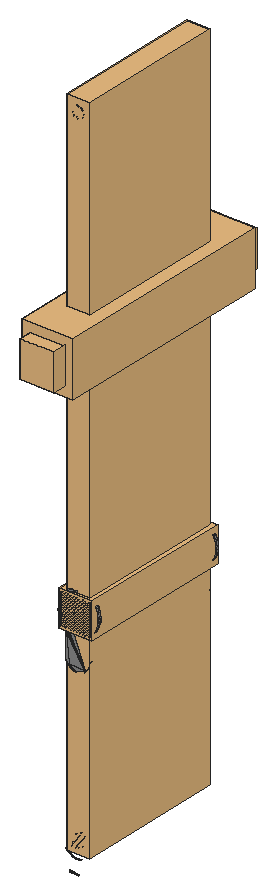
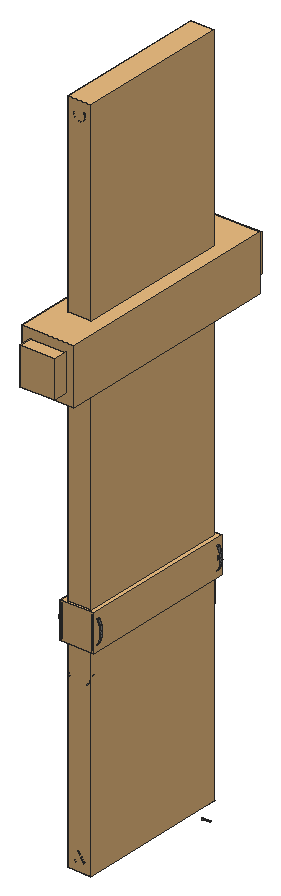
# SketchUp Ruby script. Lengths in inches.
U = 1.inch
M = Sketchup.active_model
def pt(a) = Geom::Point3d.new(a.map { |v| v * U })
def face(e, loops, mat)
  f = e.add_face(loops[0].map { |a| pt(a) })
  loops[1..].each { |l| e.add_face(l.map { |a| pt(a) }).erase! }
  f.material = f.back_material = mat if mat
  f
end
# faces: each face lists its corners as indices into pts; further lists are holes
def faces(e, pts, list, mat = nil) = list.each { |f| face(e, (f[0].is_a?(Array) ? f : [f]).map { |l| l.map { |i| pts[i] } }, mat) }
# xy, xz, yz: faces in a plane at the given z, y or x. An outline is a flat list of corners, or four numbers for a rectangle; further outlines are holes
def ring(l) = l.size == 4 ? [[l[0], l[1]], [l[2], l[1]], [l[2], l[3]], [l[0], l[3]]] : l.each_slice(2).to_a
def flat(e, list, mat, &to3) = list.each { |f| face(e, (f[0].is_a?(Array) ? f : [f]).map { |l| ring(l).map { |u, v| to3.(u, v) } }, mat) }
def xy(e, z, list, mat = nil) = flat(e, list, mat) { |x, y| [x, y, z] }
def xz(e, y, list, mat = nil) = flat(e, list, mat) { |x, z| [x, y, z] }
def yz(e, x, list, mat = nil) = flat(e, list, mat) { |y, z| [x, y, z] }
def lines(e, pts, list) = list.each { |a, b| e.add_line(pt(pts[a]), pt(pts[b])) }
# prism: a flat outline (further loops are holes) pulled along v
def prism(e, loops, v, mat = nil)
  f = face(e, loops, mat); d = Geom::Vector3d.new(v.map { |x| x * U })
  f.pushpull(f.normal.samedirection?(d) ? d.length : -d.length)
end
def box(e, o, s, mat = nil) = prism(e, [[o, [o[0] + s[0], o[1], o[2]], [o[0] + s[0], o[1] + s[1], o[2]], [o[0], o[1] + s[1], o[2]]]], [0, 0, s[2]], mat)
def at(x, y, z, deg = 0) = Geom::Transformation.translation(pt([x, y, z])) * Geom::Transformation.rotation(ORIGIN, Z_AXIS, deg.degrees)
def axes(o, x, y, z) = Geom::Transformation.new([*x, 0, *y, 0, *z, 0, *pt(o).to_a, 1])
def part(name) = M.definitions.add(name)
# library, detail: a bought-in or finely detailed component or shape, given as its bounding box
def library(name, o, s) = part(name).tap { |d| box(d.entities, o, s) }
def detail(e, o, s) = box(e.add_group.entities, o, s)
def put(e, d, t, mat = nil) = e.add_instance(d, t).tap { |i| i.material = mat if mat }
def group(e, t, mat = nil) = e.add_group.tap { |g| g.transformation = t; g.material = mat if mat }.entities
root = M.entities
M.materials.add("Material \#1").color = [140, 140, 140]
c1 = library("3DGeom~14_Defintion",[-102.17,352.37,-727.27],[204.35,204.35,1000])
c2 = library("3DGeom~4_Defintion",[-18.02,-499.97,-221.16],[36.04,1000,262.12])
c3 = part("3DGeom~5_Defintion")
xy(c3.entities,-225.24,[[-0.79,-499.98,-2.33,-499.64,7.45,-496.14],[-0.79,-499.98,7.45,-496.14,1.58,-499.88],[1.58,-499.88,7.45,-496.14,3.84,-499.16],[-2.33,-499.64,7.4,-485.75,7.45,-496.14],[3.84,-499.16,7.45,-496.14,5.85,-497.89],
  [7.45,-496.14,7.4,-485.75,8.24,-487.08],[7.45,-496.14,8.24,-487.08,8.96,-489.34],[7.45,-496.14,8.96,-489.34,9.0625,-491.71],[7.45,-496.14,9.0625,-491.71,8.55,-494.03],[-7.4,-496.08,-8.24,-494.76,2.32,-482.2],
  [-8.24,-494.76,-8.96,-492.5,2.32,-482.2],[-8.96,-492.5,-9.0625,-490.125,2.32,-482.2],[-9.0625,-490.125,-8.55,-487.81,2.32,-482.2],[-8.55,-487.81,-7.45,-485.7,2.32,-482.2],[-7.45,-485.7,-5.85,-483.95,2.32,-482.2],
  [-5.85,-483.95,-3.84,-482.68,2.32,-482.2],[-3.84,-482.68,-1.58,-481.96,2.32,-482.2],[2.32,-482.2,-1.58,-481.96,0.79,-481.86],[0,481.82,-2.35,482.13,-6.92,496.71],[0,481.82,-6.92,496.71,1.55,482.04],
  [-2.35,482.13,-4.55,483.04,-6.92,496.71],[-4.55,483.04,-6.43,484.49,-6.92,496.71],[-6.43,484.49,-7.88,486.37,-6.92,496.71],[6.92,485.12,-1.55,499.8125,7.88,495.47],[6.92,485.12,7.88,495.47,7.88,486.37],
  [-7.88,486.37,-8.79,488.57,-6.92,496.71],[7.88,486.37,7.88,495.47,8.79,488.57],[-8.79,488.57,-9.1,490.92,-6.92,496.71],[8.79,488.57,7.88,495.47,9.1,490.92],[-9.1,490.92,-8.79,493.28,-6.92,496.71],
  [9.1,490.92,7.88,495.47,8.79,493.28],[-8.79,493.28,-7.88,495.47,-6.92,496.71],[7.88,495.47,-1.55,499.8125,0,500.02],[7.88,495.47,0,500.02,2.35,499.71],[7.88,495.47,2.35,499.71,4.55,498.8],
  [7.88,495.47,4.55,498.8,6.43,497.35]],"Material \#1")
xy(c3.entities,-221.57,[[-2.33,-499.64,-5.22,-498.37,7.4,-485.75],[-5.22,-498.37,-7.4,-496.08,5.22,-483.47],[-5.22,-498.37,5.22,-483.47,7.4,-485.75],[-7.4,-496.08,2.32,-482.2,5.22,-483.47],[1.55,482.04,-6.92,496.71,-4.55,498.8],
  [1.55,482.04,-4.55,498.8,4.55,483.04],[4.55,483.04,-4.55,498.8,-1.55,499.8125],[4.55,483.04,-1.55,499.8125,6.92,485.12]],"Material \#1")
xy(c3.entities,38.05,[[-2.33,-499.64,7.4,-485.75,-5.22,-498.37],[-5.22,-498.37,5.22,-483.47,-7.4,-496.08],[-5.22,-498.37,7.4,-485.75,5.22,-483.47],[-7.4,-496.08,5.22,-483.47,2.32,-482.2],[1.55,482.04,-4.55,498.8,-6.92,496.71],
  [1.55,482.04,4.55,483.04,-4.55,498.8],[4.55,483.04,-1.55,499.8125,-4.55,498.8],[4.55,483.04,6.92,485.12,-1.55,499.8125]],"Material \#1")
xy(c3.entities,41.72,[[-0.79,-499.98,7.45,-496.14,-2.33,-499.64],[-0.79,-499.98,1.58,-499.88,7.45,-496.14],[1.58,-499.88,3.84,-499.16,7.45,-496.14],[-2.33,-499.64,7.45,-496.14,7.4,-485.75],[3.84,-499.16,5.85,-497.89,7.45,-496.14],
  [7.45,-496.14,8.24,-487.08,7.4,-485.75],[7.45,-496.14,8.55,-494.03,9.0625,-491.71],[7.45,-496.14,8.96,-489.34,8.24,-487.08],[7.45,-496.14,9.0625,-491.71,8.96,-489.34],[-7.4,-496.08,2.32,-482.2,-8.24,-494.76],
  [-8.24,-494.76,2.32,-482.2,-8.96,-492.5],[-8.96,-492.5,2.32,-482.2,-9.0625,-490.125],[-9.0625,-490.125,2.32,-482.2,-8.55,-487.81],[-8.55,-487.81,2.32,-482.2,-7.45,-485.7],[-7.45,-485.7,2.32,-482.2,-5.85,-483.95],
  [-5.85,-483.95,2.32,-482.2,-3.84,-482.68],[-3.84,-482.68,2.32,-482.2,-1.58,-481.96],[2.32,-482.2,0.79,-481.86,-1.58,-481.96],[0,481.82,-6.92,496.71,-2.35,482.13],[0,481.82,1.55,482.04,-6.92,496.71],
  [-2.35,482.13,-6.92,496.71,-4.55,483.04],[-4.55,483.04,-6.92,496.71,-6.43,484.49],[-6.43,484.49,-6.92,496.71,-7.88,486.37],[6.92,485.12,7.88,495.47,-1.55,499.8125],[6.92,485.12,7.88,486.37,7.88,495.47],
  [-7.88,486.37,-6.92,496.71,-8.79,488.57],[7.88,486.37,8.79,488.57,7.88,495.47],[-8.79,488.57,-6.92,496.71,-9.1,490.92],[8.79,488.57,9.1,490.92,7.88,495.47],[-9.1,490.92,-6.92,496.71,-8.79,493.28],
  [9.1,490.92,8.79,493.28,7.88,495.47],[-8.79,493.28,-6.92,496.71,-7.88,495.47],[7.88,495.47,0,500.02,-1.55,499.8125],[7.88,495.47,2.35,499.71,0,500.02],[7.88,495.47,4.55,498.8,2.35,499.71],
  [7.88,495.47,6.43,497.35,4.55,498.8]],"Material \#1")
c4 = library("3DGeom~1_Defintion",[-60.87,347.29,-704.08],[121.74,121.75,1000])
c5 = part("3DGeom~10_Defintion")
yz(c5.entities,-68.96,[[-797.08,-844.83,-797.08,-827.59,-922.41,-827.59],[-922.41,-844.83,-797.08,-844.83,-922.41,-827.59]],"Material \#1")
yz(c5.entities,68.97,[[-922.41,-844.83,-797.08,-827.59,-797.08,-844.83],[-922.41,-844.83,-922.41,-827.59,-797.08,-827.59],[-797.08,137.93,-922.41,155.17,-797.08,155.17],[-922.41,137.93,-922.41,155.17,-797.08,137.93]],"Material \#1")
p = [[-15.8,-989.55,-844.83],[-15.8,-989.55,-827.59],[0,-991.38,-827.59],[0,-991.38,-844.83],[15.8,-989.55,-827.59],[15.8,-989.55,-844.83],
  [-30.32,-984.36,-844.83],[-30.32,-984.36,-827.59],[30.31,-984.36,-827.59],[30.31,-984.36,-844.83],[-43.12,-976.21,-844.83],[-43.12,-976.21,-827.59],
  [43.12,-976.21,-827.59],[43.12,-976.21,-844.83],[-53.81,-965.53,-844.83],[-53.81,-965.53,-827.59],[53.8,-965.53,-827.59],[53.8,-965.53,-844.83],
  [-61.95,-952.73,-844.83],[-61.95,-952.73,-827.59],[53.8,-965.53,-827.59],[61.95,-952.73,-827.59],[61.95,-952.73,-844.83],[-67.15,-938.21,-844.83],
  [-67.15,-938.21,-827.59],[67.14,-938.21,-827.59],[67.14,-938.21,-844.83],[-68.96,-922.41,-844.83],[-68.96,-922.41,-827.59],[67.14,-938.21,-827.59],
  [68.97,-922.41,-827.59],[68.97,-922.41,-844.83],[-69.1,-794.86,-844.83],[-69.1,-794.86,-827.59],[-68.96,-797.08,-827.59],[-68.96,-797.08,-844.83],
  [68.97,-797.08,-844.83],[68.97,-797.08,-827.59],[69.11,-794.71,-827.59],[69.11,-794.71,-844.83],[-69.48,-792.73,-844.83],[-69.48,-792.73,-827.59],
  [69.53,-792.51,-827.59],[69.53,-792.51,-844.83],[-70.14,-790.6875,-844.83],[-70.14,-790.6875,-827.59],[70.24,-790.48,-827.59],[70.24,-790.48,-844.83],
  [-71.08,-788.73,-844.83],[-71.08,-788.73,-827.59],[71.22,-788.57,-827.59],[71.22,-788.57,-844.83],[-72.32,-786.86,-844.83],[-72.32,-786.86,-827.59],
  [72.47,-786.78,-827.59],[72.47,-786.78,-844.83],[-73.8,-785.17,-844.83],[-73.8,-785.17,-827.59],[74,-785.04,-827.59],[74,-785.04,-844.83],
  [-75.96,-783.21,-844.83],[-75.96,-783.21,-827.59],[74,-785.04,-827.59],[75.76,-783.39,-827.59],[75.76,-783.39,-844.83],[86.625,-772.95,-827.59],
  [86.61,-772.96,-844.83],[-86.89,-773.25,-844.83],[-86.89,-773.25,-827.59],[-75.96,-783.21,-844.83],[-96.66,-761.8,-844.83],[-96.66,-761.8,-827.59],
  [86.625,-772.95,-827.59],[86.63,-772.94,-844.83],[86.61,-772.96,-844.83],[86.625,-772.95,-827.59],[86.62,-772.95,-827.59],[86.62,-772.95,-827.59],
  [96.31,-761.375,-827.59],[96.31,-761.375,-844.83],[86.63,-772.94,-844.83],[86.625,-772.95,-827.59],[86.62,-772.95,-827.59],[-104.96,-749.18,-844.83],
  [-104.96,-749.18,-827.59],[-96.66,-761.8,-827.59],[-96.66,-761.8,-844.83],[96.31,-761.375,-827.59],[104.62,-748.77,-827.59],[104.62,-748.77,-844.83],
  [-111.64,-735.52,-844.83],[-111.64,-735.52,-827.59],[111.39,-735.21,-827.59],[111.39,-735.21,-844.83],[-116.49,-721.23,-844.83],[-116.49,-721.23,-827.59],
  [116.4375,-720.78,-827.59],[116.4375,-720.78,-844.83],[-119.64,-705.62,-844.83],[-119.64,-705.62,-827.59],[119.6,-705.57,-827.59],[119.6,-705.57,-844.83],
  [-120.6875,-689.65,-844.83],[-120.6875,-689.65,-827.59],[120.69,-689.65,-827.59],[120.69,-689.65,-844.83],[-117.5,-662,-844.83],[-117.5,-662,-827.59],
  [117.5,-662,-827.59],[117.5,-662,-844.83],[-108.41,-636.61,-844.83],[-108.41,-636.61,-827.59],[117.5,-662,-844.83],[108.41,-636.61,-827.59],
  [108.41,-636.61,-844.83],[-93.91,-613.95,-844.83],[-93.91,-613.95,-827.59],[-108.41,-636.61,-827.59],[108.41,-636.61,-844.83],[94.16,-614.19,-827.59],
  [94.16,-614.19,-844.83],[94.16,-614.19,-827.59],[75.46,-595.5,-827.59],[75.46,-595.5,-844.83],[-75.46,-595.5,-844.83],[-75.46,-595.5,-827.59],
  [-93.91,-613.95,-827.59],[-93.91,-613.95,-827.59],[-93.91,-613.95,-844.83],[-53.05,-581.24,-844.83],[-53.05,-581.24,-827.59],[-75.46,-595.5,-827.59],
  [-75.46,-595.5,-844.83],[53.05,-581.24,-827.59],[53.05,-581.24,-844.83],[-27.65,-572.16,-844.83],[-27.65,-572.16,-827.59],[-53.05,-581.24,-827.59],
  [-53.05,-581.24,-844.83],[27.66,-572.16,-827.59],[27.66,-572.16,-844.83],[0,-568.97,-844.83],[0,-568.97,-827.59],[-27.65,-572.16,-827.59],
  [-27.65,-572.16,-844.83],[0,-568.97,-844.83],[-15.8,-989.55,155.17],[0,-991.38,155.17],[0,-991.38,137.93],[-15.8,-989.55,137.93],
  [15.8,-989.55,155.17],[15.8,-989.55,137.93],[-30.32,-984.36,155.17],[-30.32,-984.36,137.93],[30.31,-984.36,155.17],[30.31,-984.36,137.93],
  [-43.125,-976.22,155.17],[-43.125,-976.22,137.93],[43.12,-976.22,155.17],[43.12,-976.22,137.93],[-53.81,-965.53,155.17],[-53.81,-965.53,137.93],
  [53.8,-965.53,155.17],[53.8,-965.53,137.93],[-61.96,-952.73,155.17],[-61.95,-952.73,137.93],[61.95,-952.73,155.17],[61.95,-952.73,137.93],
  [53.8,-965.53,137.93],[-67.15,-938.21,155.17],[-67.15,-938.21,137.93],[67.14,-938.21,155.17],[67.14,-938.21,137.93],[-68.96,-922.41,155.17],
  [-68.96,-922.41,137.93],[68.97,-922.41,155.17],[68.97,-922.41,137.93],[67.14,-938.21,137.93],[-68.97,-797.08,155.17],[-68.97,-797.08,137.93],
  [-69.1,-794.86,155.17],[-69.1,-794.86,137.93],[68.97,-797.08,155.17],[69.11,-794.71,155.17],[69.11,-794.71,137.93],[68.97,-797.08,137.93],
  [-69.48,-792.73,155.17],[-69.48,-792.73,137.93],[69.53,-792.51,155.17],[69.53,-792.51,137.93],[-70.14,-790.6875,155.17],[-70.14,-790.6875,137.93],
  [70.24,-790.48,155.17],[70.24,-790.48,137.93],[-71.08,-788.73,155.17],[-71.08,-788.73,137.93],[71.22,-788.57,155.17],[71.22,-788.57,137.93],
  [-72.32,-786.86,155.17],[-72.32,-786.86,137.93],[72.47,-786.78,155.17],[72.47,-786.78,137.93],[-73.8,-785.17,155.17],[-73.8,-785.17,137.93],
  [74,-785.04,155.17],[74,-785.04,137.93],[-75.96,-783.21,155.17],[-75.96,-783.21,137.93],[75.76,-783.39,155.17],[75.76,-783.39,137.93],
  [74,-785.04,137.93],[86.61,-772.96,155.17],[86.625,-772.95,137.93],[-86.88,-773.25,155.17],[-75.96,-783.21,155.17],[-86.88,-773.25,137.93],
  [-96.66,-761.8,155.17],[-96.66,-761.8,137.93],[86.63,-772.94,155.17],[86.625,-772.95,137.93],[86.61,-772.96,155.17],[86.62,-772.95,137.93],
  [86.625,-772.95,137.93],[96.31,-761.375,155.17],[96.31,-761.375,137.93],[86.62,-772.95,137.93],[86.63,-772.94,155.17],[86.62,-772.95,137.93],
  [86.625,-772.95,137.93],[-104.96,-749.18,155.17],[-96.66,-761.8,155.17],[-96.66,-761.8,137.93],[-104.96,-749.18,137.93],[104.62,-748.77,155.17],
  [104.62,-748.77,137.93],[96.31,-761.375,137.93],[-111.64,-735.52,155.17],[-111.64,-735.52,137.93],[111.39,-735.21,155.17],[111.39,-735.21,137.93],
  [-116.49,-721.23,155.17],[-116.49,-721.23,137.93],[116.4375,-720.78,155.17],[116.4375,-720.78,137.93],[-119.64,-705.62,155.17],[-119.64,-705.62,137.93],
  [119.6,-705.57,155.17],[119.6,-705.57,137.93],[-120.6875,-689.65,155.17],[-120.6875,-689.65,137.93],[120.69,-689.65,155.17],[120.69,-689.65,137.93],
  [-117.5,-662,155.17],[-117.5,-662,137.93],[117.5,-662,155.17],[117.5,-662,137.93],[-108.41,-636.61,155.17],[-108.41,-636.61,137.93],
  [117.5,-662,155.17],[108.41,-636.61,155.17],[108.41,-636.61,137.93],[-93.91,-613.95,155.17],[-108.41,-636.61,137.93],[-93.91,-613.95,137.93],
  [108.41,-636.61,155.17],[94.16,-614.19,155.17],[94.16,-614.19,137.93],[75.46,-595.5,155.17],[75.46,-595.5,137.93],[94.16,-614.19,137.93],
  [-75.46,-595.5,155.17],[-93.91,-613.95,155.17],[-93.91,-613.95,137.93],[-75.46,-595.5,137.93],[-53.05,-581.24,155.17],[-75.46,-595.5,155.17],
  [-75.46,-595.5,137.93],[-53.05,-581.24,137.93],[53.05,-581.24,155.17],[53.05,-581.24,137.93],[-27.65,-572.16,155.17],[-53.05,-581.24,155.17],
  [-53.05,-581.24,137.93],[-27.65,-572.16,137.93],[27.65,-572.16,155.17],[27.65,-572.16,137.93],[0,-568.97,155.17],[-27.65,-572.16,155.17],
  [-27.65,-572.16,137.93],[0,-568.97,137.93],[0,-568.97,155.17]]
faces(c5.entities,p,[[0,1,2],[2,3,0],[3,2,4],[4,5,3],[6,7,1],[1,0,6],[5,4,8],[8,9,5],
  [10,11,7],[7,6,10],[9,8,12],[12,13,9],[14,15,11],[11,10,14],[13,12,16],[16,17,13],
  [18,19,15],[15,14,18],[17,20,21],[21,22,17],[23,24,19],[19,18,23],[22,21,25],[25,26,22],
  [27,28,24],[24,23,27],[26,29,30],[30,31,26],[32,33,34],[34,35,32],[36,37,38],[38,39,36],
  [40,41,33],[33,32,40],[39,38,42],[42,43,39],[44,45,41],[41,40,44],[43,42,46],[46,47,43],
  [48,49,45],[45,44,48],[47,46,50],[50,51,47],[52,53,49],[49,48,52],[51,50,54],[54,55,51],
  [56,57,53],[53,52,56],[55,54,58],[58,59,55],[60,61,57],[57,56,60],[59,62,63],[63,64,59],
  [64,63,65],[65,66,64],[67,68,61],[61,69,67],[70,71,68],[68,67,70],[72,73,66],[74,75,76],
  [73,77,78],[78,79,73],[80,81,82],[83,84,85],[85,86,83],[79,87,88],[88,89,79],[90,91,84],
  [84,83,90],[89,88,92],[92,93,89],[94,95,91],[91,90,94],[93,92,96],[96,97,93],[98,99,95],
  [95,94,98],[97,96,100],[100,101,97],[102,103,99],[99,98,102],[101,100,104],[104,105,101],[106,107,103],
  [103,102,106],[105,104,108],[108,109,105],[110,111,107],[107,106,110],[112,108,113],[113,114,112],[115,116,117],
  [117,110,115],[118,113,119],[119,120,118],[120,121,122],[122,123,120],[124,125,126],[127,128,124],[129,130,131],
  [131,132,129],[123,122,133],[133,134,123],[135,136,137],[137,138,135],[134,133,139],[139,140,134],[141,142,143],
  [143,144,141],[140,139,142],[142,145,140],[146,147,148],[148,149,146],[147,150,151],[151,148,147],[152,146,149],
  [149,153,152],[150,154,155],[155,151,150],[156,152,153],[153,157,156],[154,158,159],[159,155,154],[160,156,157],
  [157,161,160],[158,162,163],[163,159,158],[164,160,161],[161,165,164],[162,166,167],[167,168,162],[169,164,165],
  [165,170,169],[166,171,172],[172,167,166],[173,169,170],[170,174,173],[171,175,176],[176,177,171],[178,173,174],
  [174,179,178],[180,178,179],[179,181,180],[182,183,184],[184,185,182],[186,180,181],[181,187,186],[183,188,189],
  [189,184,183],[190,186,187],[187,191,190],[188,192,193],[193,189,188],[194,190,191],[191,195,194],[192,196,197],
  [197,193,192],[198,194,195],[195,199,198],[196,200,201],[201,197,196],[202,198,199],[199,203,202],[200,204,205],
  [205,201,200],[206,202,203],[203,207,206],[204,208,209],[209,210,204],[208,211,212],[212,209,208],[213,214,207],
  [207,215,213],[216,213,215],[215,217,216],[211,218,219],[220,221,222],[218,223,224],[224,225,218],[226,227,228],
  [229,230,231],[231,232,229],[223,233,234],[234,235,223],[236,229,232],[232,237,236],[233,238,239],[239,234,233],
  [240,236,237],[237,241,240],[238,242,243],[243,239,238],[244,240,241],[241,245,244],[242,246,247],[247,243,242],
  [248,244,245],[245,249,248],[246,250,251],[251,247,246],[252,248,249],[249,253,252],[250,254,255],[255,251,250],
  [256,252,253],[253,257,256],[258,259,260],[260,255,258],[261,256,262],[262,263,261],[264,265,266],[266,260,264],
  [265,267,268],[268,269,265],[270,271,272],[272,273,270],[274,275,276],[276,277,274],[267,278,279],[279,268,267],
  [280,281,282],[282,283,280],[278,284,285],[285,279,278],[286,287,288],[288,289,286],[284,290,289],[289,285,284]],"Material \#1")
c6 = library("3DGeom~12_Defintion",[-95.68,-755.75,-830.03],[191.36,191.37,1000])
c7 = library("3DGeom~13_Defintion",[-84.91,-744.98,-830.03],[169.82,169.83,1000])
xy(root,161.124,[[359.541,199.268,359.541,199.557,359.571,199.557],[359.541,199.268,359.571,199.557,359.571,199.268]],"Material \#1")
xy(root,161.418,[[359.526,199.268,359.576,199.268,359.526,199.557],[359.576,199.268,359.576,199.557,359.526,199.557]],"Material \#1")
xz(root,199.268,[[359.551,161.075,359.503,161.081,359.551,161.082],[359.551,161.075,359.551,161.082,359.597,161.088],[359.551,161.075,359.597,161.088,359.599,161.081],[359.503,161.081,359.459,161.101,359.505,161.088],[359.503,161.081,359.505,161.088,359.551,161.082],
  [359.599,161.081,359.597,161.088,359.64,161.107],[359.599,161.081,359.64,161.107,359.644,161.101],[359.505,161.088,359.459,161.101,359.462,161.107],[359.459,161.101,359.421,161.132,359.462,161.107],[359.644,161.101,359.64,161.107,359.677,161.137],
  [359.644,161.101,359.677,161.137,359.682,161.132],[359.462,161.107,359.421,161.132,359.426,161.137],[359.421,161.132,359.391,161.173,359.426,161.137],[359.682,161.132,359.677,161.137,359.705,161.176],[359.682,161.132,359.705,161.176,359.711,161.173],
  [359.426,161.137,359.391,161.173,359.397,161.176],[359.391,161.173,359.373,161.22,359.397,161.176],[359.711,161.173,359.705,161.176,359.723,161.222],[359.711,161.173,359.723,161.222,359.73,161.22],[359.397,161.176,359.373,161.22,359.38,161.222],
  [359.373,161.22,359.367,161.271,359.38,161.222],[359.73,161.22,359.723,161.222,359.729,161.271],[359.73,161.22,359.729,161.271,359.736,161.271],[359.38,161.222,359.367,161.271,359.374,161.271],[359.367,161.271,359.373,161.322,359.374,161.271],
  [359.374,161.271,359.373,161.322,359.38,161.32],[359.729,161.271,359.723,161.32,359.736,161.271],[359.736,161.271,359.723,161.32,359.73,161.322],[359.38,161.32,359.373,161.322,359.391,161.369],[359.38,161.32,359.391,161.369,359.397,161.366],
  [359.723,161.32,359.705,161.366,359.73,161.322],[359.73,161.322,359.705,161.366,359.711,161.369],[359.397,161.366,359.391,161.369,359.421,161.41],[359.397,161.366,359.421,161.41,359.426,161.405],[359.705,161.366,359.677,161.405,359.711,161.369],
  [359.711,161.369,359.677,161.405,359.682,161.41],[359.426,161.405,359.421,161.41,359.459,161.441],[359.426,161.405,359.459,161.441,359.462,161.435],[359.677,161.405,359.64,161.435,359.682,161.41],[359.682,161.41,359.64,161.435,359.644,161.441],
  [359.462,161.435,359.459,161.441,359.503,161.461],[359.462,161.435,359.503,161.461,359.505,161.454],[359.64,161.435,359.597,161.454,359.644,161.441],[359.644,161.441,359.597,161.454,359.599,161.461],[359.505,161.454,359.503,161.461,359.551,161.467],
  [359.505,161.454,359.551,161.467,359.551,161.46],[359.597,161.454,359.551,161.46,359.599,161.461],[359.551,161.46,359.551,161.467,359.599,161.461]],"Material \#1")
xz(root,199.277,[[359.551,160.635,359.449,160.688,359.654,160.688],[359.551,160.635,359.494,160.65,359.449,160.688],[359.551,160.635,359.521,160.639,359.494,160.65],[359.494,160.65,359.469,160.666,359.449,160.688],[359.654,160.688,359.318,161.238,359.39,161.133],
  [359.654,160.688,359.415,161.063,359.318,161.238],[359.449,160.688,359.42,161.042,359.42,161.048],[359.449,160.688,359.42,161.048,359.654,160.688],[359.449,160.688,359.423,160.743,359.42,161.042],[359.449,160.688,359.433,160.714,359.423,160.743],
  [359.654,160.688,359.46,161.073,359.504,161.056],[359.423,160.743,359.42,160.775,359.42,161.042],[359.368,161.427,359.448,161.495,359.551,161.521],[359.368,161.427,359.551,161.521,359.46,161.469],[359.46,161.469,359.551,161.521,359.504,161.486],
  [359.504,161.486,359.551,161.521,359.551,161.491],[359.448,161.495,359.497,161.514,359.551,161.521]],"Material \#1")
xz(root,199.308,[[359.551,158.424,359.443,158.434,359.551,158.435],[359.443,158.434,359.444,158.445,359.551,158.435],[359.551,158.596,359.515,158.599,359.551,158.607],[359.551,158.596,359.551,158.607,359.585,158.61],[359.515,158.599,359.481,158.609,359.517,158.61],
  [359.515,158.599,359.517,158.61,359.551,158.607],[359.481,158.609,359.45,158.625,359.485,158.62],[359.481,158.609,359.485,158.62,359.517,158.61],[359.485,158.62,359.45,158.625,359.455,158.635],[359.45,158.625,359.422,158.646,359.455,158.635],
  [359.455,158.635,359.422,158.646,359.429,158.655],[359.422,158.646,359.398,158.672,359.429,158.655],[359.406,158.94,359.422,158.973,359.429,158.964],[359.429,158.964,359.422,158.973,359.45,158.994],[359.429,158.964,359.45,158.994,359.455,158.984],
  [359.455,158.984,359.45,158.994,359.481,159.01],[359.455,158.984,359.481,159.01,359.485,158.999],[359.485,158.999,359.481,159.01,359.515,159.019],[359.485,158.999,359.515,159.019,359.517,159.009],[359.517,159.009,359.515,159.019,359.551,159.023],
  [359.517,159.009,359.551,159.023,359.551,159.012],[359.551,159.012,359.551,159.023,359.587,159.019]],"Material \#1")
xz(root,199.339,[[359.551,161.051,359.498,161.058,359.551,161.058],[359.551,161.051,359.551,161.058,359.603,161.065],[359.551,161.051,359.603,161.065,359.605,161.058],[359.498,161.058,359.448,161.08,359.499,161.065],[359.498,161.058,359.499,161.065,359.551,161.058],
  [359.605,161.058,359.603,161.065,359.651,161.087],[359.605,161.058,359.651,161.087,359.655,161.08],[359.499,161.065,359.448,161.08,359.451,161.087],[359.448,161.08,359.405,161.115,359.451,161.087],[359.655,161.08,359.651,161.087,359.693,161.12],
  [359.655,161.08,359.693,161.12,359.698,161.115],[359.451,161.087,359.405,161.115,359.41,161.12],[359.405,161.115,359.372,161.161,359.41,161.12],[359.698,161.115,359.693,161.12,359.725,161.165],[359.698,161.115,359.725,161.165,359.731,161.161],
  [359.41,161.12,359.372,161.161,359.378,161.165],[359.372,161.161,359.351,161.214,359.378,161.165],[359.731,161.161,359.725,161.165,359.745,161.216],[359.731,161.161,359.745,161.216,359.751,161.214],[359.378,161.165,359.351,161.214,359.358,161.216],
  [359.351,161.214,359.344,161.271,359.358,161.216],[359.751,161.214,359.745,161.216,359.751,161.271],[359.751,161.214,359.751,161.271,359.758,161.271],[359.358,161.216,359.344,161.271,359.351,161.271],[359.344,161.271,359.351,161.328,359.351,161.271],
  [359.351,161.271,359.351,161.328,359.358,161.326],[359.751,161.271,359.745,161.326,359.758,161.271],[359.758,161.271,359.745,161.326,359.751,161.328],[359.358,161.326,359.351,161.328,359.372,161.381],[359.358,161.326,359.372,161.381,359.378,161.378],
  [359.745,161.326,359.725,161.378,359.751,161.328],[359.751,161.328,359.725,161.378,359.731,161.381],[359.378,161.378,359.372,161.381,359.405,161.427],[359.378,161.378,359.405,161.427,359.41,161.422],[359.725,161.378,359.693,161.422,359.731,161.381],
  [359.731,161.381,359.693,161.422,359.698,161.427],[359.41,161.422,359.405,161.427,359.448,161.462],[359.41,161.422,359.448,161.462,359.451,161.456],[359.693,161.422,359.651,161.456,359.698,161.427],[359.698,161.427,359.651,161.456,359.655,161.462],
  [359.451,161.456,359.448,161.462,359.498,161.484],[359.451,161.456,359.498,161.484,359.499,161.477],[359.651,161.456,359.603,161.477,359.655,161.462],[359.655,161.462,359.603,161.477,359.605,161.484],[359.499,161.477,359.498,161.484,359.551,161.491],
  [359.499,161.477,359.551,161.491,359.551,161.484],[359.603,161.477,359.551,161.484,359.605,161.484],[359.551,161.484,359.551,161.491,359.605,161.484]],"Material \#1")
xz(root,199.557,[[359.541,161.124,359.531,161.146,359.561,161.146],[359.541,161.124,359.561,161.146,359.571,161.124],[359.531,161.146,359.526,161.153,359.567,161.153],[359.531,161.146,359.567,161.153,359.561,161.146],[359.526,161.153,359.526,161.17,359.567,161.17],
  [359.526,161.153,359.567,161.17,359.567,161.153],[359.526,161.17,359.531,161.177,359.561,161.177],[359.526,161.17,359.561,161.177,359.567,161.17],[359.531,161.177,359.531,161.205,359.571,161.205],[359.531,161.177,359.571,161.205,359.561,161.177],
  [359.531,161.205,359.531,161.231,359.571,161.231],[359.531,161.205,359.571,161.231,359.571,161.205],[359.531,161.231,359.524,161.251,359.579,161.251],[359.531,161.231,359.579,161.251,359.571,161.231],[359.524,161.251,359.524,161.272,359.579,161.272],
  [359.524,161.251,359.579,161.272,359.579,161.251],[359.524,161.272,359.531,161.293,359.571,161.293],[359.524,161.272,359.571,161.293,359.579,161.272],[359.531,161.293,359.526,161.308,359.576,161.308],[359.531,161.293,359.576,161.308,359.571,161.293],
  [359.526,161.308,359.526,161.356,359.576,161.356],[359.526,161.308,359.576,161.356,359.576,161.308],[359.526,161.356,359.533,161.359,359.57,161.359],[359.526,161.356,359.57,161.359,359.576,161.356],[359.533,161.359,359.533,161.367,359.57,161.367],
  [359.533,161.359,359.57,161.367,359.57,161.359],[359.533,161.367,359.526,161.37,359.576,161.37],[359.533,161.367,359.576,161.37,359.57,161.367],[359.526,161.37,359.526,161.418,359.576,161.418],[359.526,161.37,359.576,161.418,359.576,161.37]],"Material \#1")
xz(root,199.588,[[359.551,160.635,359.494,160.65,359.521,160.639],[359.551,160.635,359.609,160.65,359.494,160.65],[359.494,160.65,359.42,161.042,359.423,160.743],[359.494,160.65,359.679,160.743,359.42,161.042],[359.494,160.65,359.423,160.743,359.449,160.688],
  [359.494,160.65,359.449,160.688,359.469,160.666],[359.449,160.688,359.423,160.743,359.433,160.714],[359.679,160.743,359.415,161.063,359.417,161.058],[359.679,160.743,359.417,161.058,359.419,161.053],[359.679,160.743,359.419,161.053,359.42,161.048],
  [359.423,160.743,359.42,161.042,359.42,160.775],[359.679,160.743,359.42,161.048,359.42,161.042],[359.682,160.775,359.39,161.133,359.415,161.063],[359.682,160.775,359.422,161.099,359.39,161.133],[359.682,160.775,359.46,161.073,359.422,161.099],
  [359.682,160.775,359.504,161.056,359.46,161.073],[359.368,161.427,359.422,161.443,359.46,161.469],[359.368,161.427,359.46,161.469,359.551,161.521],[359.368,161.427,359.551,161.521,359.448,161.495],[359.46,161.469,359.504,161.486,359.551,161.521],
  [359.504,161.486,359.551,161.491,359.551,161.521],[359.448,161.495,359.551,161.521,359.497,161.514]],"Material \#1")
xz(root,200.833,[[359.368,161.427,359.448,161.495,359.551,161.521],[359.368,161.427,359.551,161.521,359.46,161.469],[359.504,161.486,359.551,161.521,359.551,161.491]],"Material \#1")
yz(root,359.526,[[199.557,161.37,199.268,161.418,199.557,161.418]],"Material \#1")
yz(root,359.531,[[199.557,161.177,199.268,161.205,199.557,161.205]],"Material \#1")
p = [[359.496,199.305,158.768],[359.496,199.33,158.768],[359.482,199.333,158.748],[359.482,199.308,158.748],[359.467,199.34,158.725],[359.467,199.315,158.725],
  [359.484,199.34,158.708],[359.484,199.315,158.708],[359.505,199.34,158.696],[359.505,199.315,158.696],[359.52,199.333,158.719],[359.52,199.308,158.719],
  [359.534,199.33,158.74],[359.534,199.305,158.74],[359.607,199.33,158.851],[359.607,199.305,158.851],[359.569,199.305,158.879],[359.569,199.33,158.879],
  [359.621,199.333,158.871],[359.621,199.308,158.871],[359.636,199.34,158.894],[359.636,199.315,158.894],[359.618,199.34,158.911],[359.618,199.315,158.911],
  [359.597,199.34,158.923],[359.597,199.315,158.923],[359.582,199.333,158.9],[359.582,199.308,158.9],[359.526,199.557,161.153],[359.529,199.268,161.15],
  [359.529,199.268,161.174],[359.529,199.268,161.15],[359.526,199.557,161.153],[359.531,199.557,161.146],[359.529,199.268,161.15],[359.531,199.557,161.146],
  [359.541,199.557,161.124],[359.541,199.268,161.124],[359.529,199.268,161.15],[359.531,199.557,161.177],[359.529,199.268,161.174],[359.531,199.268,161.205],
  [359.531,199.557,161.231],[359.528,199.268,161.241],[359.524,199.268,161.262],[359.531,199.557,161.205],[359.531,199.268,161.205],[359.528,199.268,161.241],
  [359.526,199.557,161.17],[359.529,199.268,161.174],[359.531,199.557,161.177],[359.526,199.557,161.17],[359.524,199.268,161.262],[359.524,199.557,161.251],
  [359.531,199.557,161.231],[359.528,199.268,161.241],[359.531,199.557,161.231],[359.531,199.557,161.205],[359.524,199.557,161.251],[359.524,199.268,161.262],
  [359.528,199.268,161.283],[359.526,199.557,161.308],[359.527,199.268,161.311],[359.529,199.268,161.36],[359.531,199.557,161.293],[359.529,199.268,161.3],
  [359.527,199.268,161.311],[359.524,199.557,161.272],[359.528,199.268,161.283],[359.529,199.268,161.3],[359.529,199.268,161.36],[359.526,199.557,161.356],
  [359.526,199.557,161.308],[359.527,199.268,161.311],[359.526,199.557,161.308],[359.531,199.557,161.293],[359.529,199.268,161.3],[359.531,199.557,161.293],
  [359.524,199.557,161.272],[359.528,199.268,161.283],[359.524,199.557,161.272],[359.524,199.557,161.251],[359.526,199.557,161.37],[359.529,199.268,161.36],
  [359.526,199.268,161.418],[359.529,199.268,161.36],[359.533,199.557,161.367],[359.533,199.557,161.359],[359.529,199.268,161.36],[359.526,199.557,161.37],
  [359.529,199.268,161.36],[359.526,199.557,161.356],[359.574,199.268,161.364],[359.576,199.557,161.356],[359.57,199.557,161.359],[359.574,199.268,161.364],
  [359.57,199.557,161.367],[359.576,199.557,161.37],[359.574,199.268,161.364]]
faces(root,p,[[0,1,2],[2,3,0],[3,2,4],[4,5,3],[5,4,6],[6,7,5],[7,6,8],[8,9,7],
  [9,8,10],[10,11,9],[11,10,12],[12,13,11],[13,12,14],[14,15,13],[16,17,1],[1,0,16],
  [15,14,18],[18,19,15],[19,18,20],[20,21,19],[21,20,22],[22,23,21],[23,22,24],[24,25,23],
  [25,24,26],[26,27,25],[27,26,17],[17,16,27],[28,29,30],[31,32,33],[34,35,36],[36,37,38],
  [39,40,41],[42,43,44],[45,46,47],[30,48,28],[49,50,51],[52,53,54],[55,56,57],[58,59,60],
  [61,62,63],[64,65,66],[67,68,69],[70,71,72],[73,74,75],[76,77,78],[79,80,81],[82,83,84],
  [85,86,87],[88,89,86],[90,87,91],[92,93,94],[95,96,97],[98,94,96]],"Material \#1")
put(root,c1,axes([359.55,200.83,162.74],[0.00304,0,0],[0,0,0.00323],[0,0.00274,0]),"Material \#1")
put(root,c2,axes([359.55,200.83,162.74],[0.00767,0,0],[0,0,0.00816],[0,0.00691,0]),"Material \#1")
put(root,c3,axes([359.55,200.83,162.74],[0.00753,0,0],[0,0,0.00801],[0,0.00678,0]),"Material \#1")
put(root,c4,axes([359.55,200.83,162.74],[0.00338,0,0],[0,0,0.0036],[0,0.00305,0]),"Material \#1")
put(root,c5,axes([359.55,200.83,162.74],[0.002,0,0],[0,0,0.00213],[0,0.0018,0]),"Material \#1")
put(root,c6,axes([359.55,200.83,162.74],[0.00209,0,0],[0,0,0.00223],[0,0.00189,0]),"Material \#1")
put(root,c7,axes([359.55,200.83,162.74],[0.00209,0,0],[0,0,0.00223],[0,0.00189,0]),"Material \#1")
